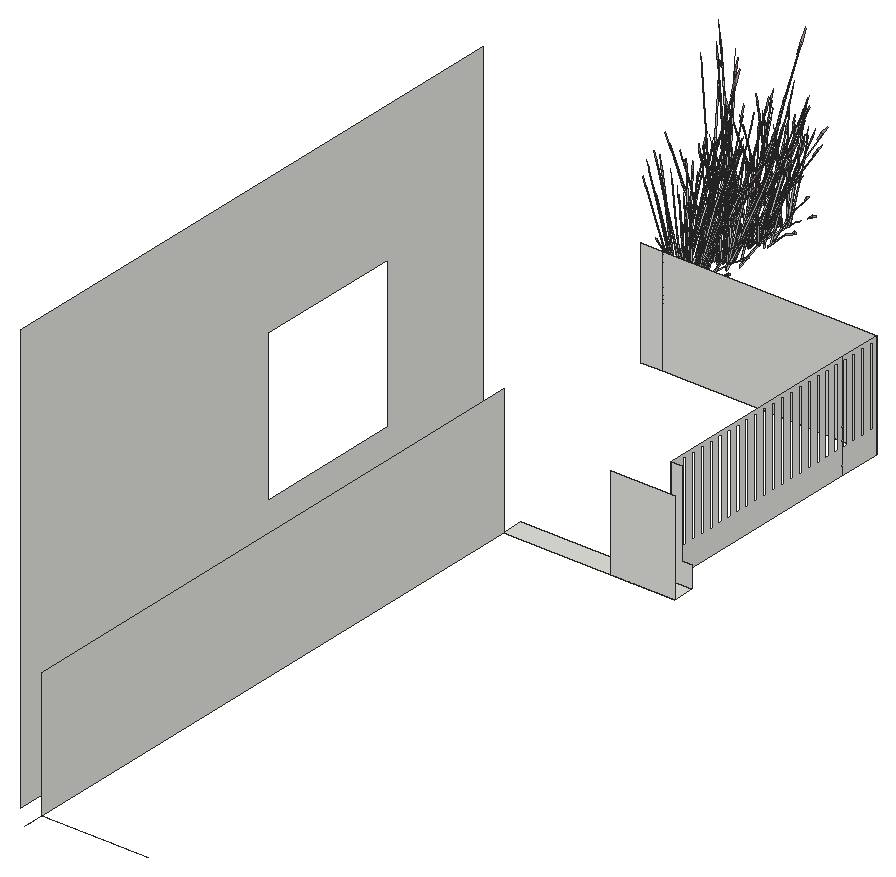
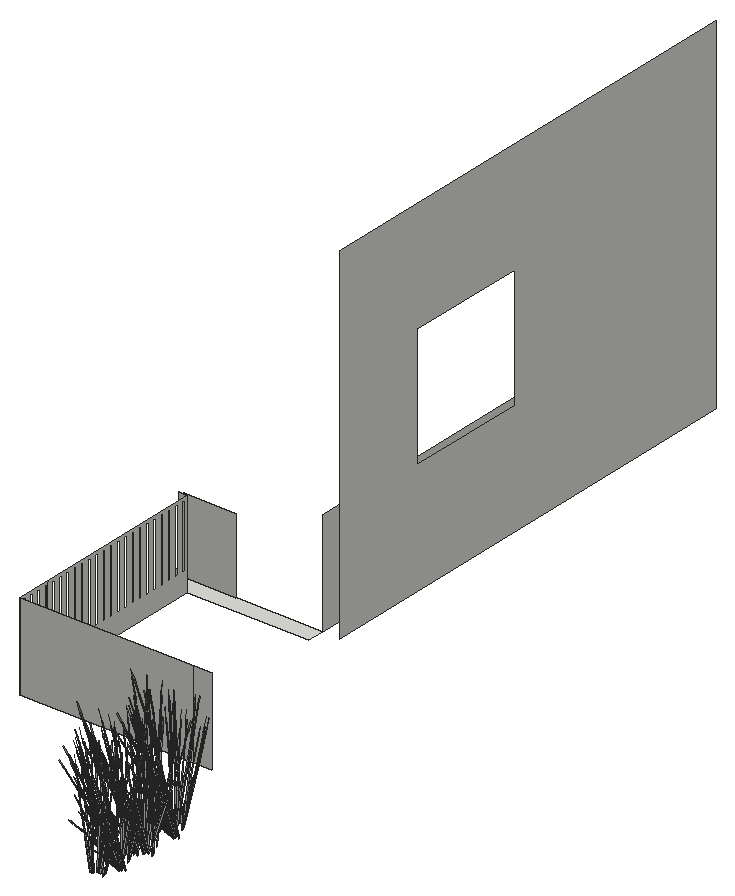
# SketchUp Ruby script. Lengths in inches.
U = 1.inch
M = Sketchup.active_model
def pt(a) = Geom::Point3d.new(a.map { |v| v * U })
def face(e, loops, mat)
  f = e.add_face(loops[0].map { |a| pt(a) })
  loops[1..].each { |l| e.add_face(l.map { |a| pt(a) }).erase! }
  f.material = f.back_material = mat if mat
  f
end
# faces: each face lists its corners as indices into pts; further lists are holes
def faces(e, pts, list, mat = nil) = list.each { |f| face(e, (f[0].is_a?(Array) ? f : [f]).map { |l| l.map { |i| pts[i] } }, mat) }
# xy, xz, yz: faces in a plane at the given z, y or x. An outline is a flat list of corners, or four numbers for a rectangle; further outlines are holes
def ring(l) = l.size == 4 ? [[l[0], l[1]], [l[2], l[1]], [l[2], l[3]], [l[0], l[3]]] : l.each_slice(2).to_a
def flat(e, list, mat, &to3) = list.each { |f| face(e, (f[0].is_a?(Array) ? f : [f]).map { |l| ring(l).map { |u, v| to3.(u, v) } }, mat) }
def xy(e, z, list, mat = nil) = flat(e, list, mat) { |x, y| [x, y, z] }
def xz(e, y, list, mat = nil) = flat(e, list, mat) { |x, z| [x, y, z] }
def yz(e, x, list, mat = nil) = flat(e, list, mat) { |y, z| [x, y, z] }
def lines(e, pts, list) = list.each { |a, b| e.add_line(pt(pts[a]), pt(pts[b])) }
# prism: a flat outline (further loops are holes) pulled along v
def prism(e, loops, v, mat = nil)
  f = face(e, loops, mat); d = Geom::Vector3d.new(v.map { |x| x * U })
  f.pushpull(f.normal.samedirection?(d) ? d.length : -d.length)
end
def box(e, o, s, mat = nil) = prism(e, [[o, [o[0] + s[0], o[1], o[2]], [o[0] + s[0], o[1] + s[1], o[2]], [o[0], o[1] + s[1], o[2]]]], [0, 0, s[2]], mat)
def at(x, y, z, deg = 0) = Geom::Transformation.translation(pt([x, y, z])) * Geom::Transformation.rotation(ORIGIN, Z_AXIS, deg.degrees)
def axes(o, x, y, z) = Geom::Transformation.new([*x, 0, *y, 0, *z, 0, *pt(o).to_a, 1])
def part(name) = M.definitions.add(name)
# library, detail: a bought-in or finely detailed component or shape, given as its bounding box
def library(name, o, s) = part(name).tap { |d| box(d.entities, o, s) }
def detail(e, o, s) = box(e.add_group.entities, o, s)
def put(e, d, t, mat = nil) = e.add_instance(d, t).tap { |i| i.material = mat if mat }
def group(e, t, mat = nil) = e.add_group.tap { |g| g.transformation = t; g.material = mat if mat }.entities
root = M.entities
M.materials.add("LightPink_Translucent").color = [144, 107, 117]
M.materials["LightPink_Translucent"].alpha = 0.75
c1 = part("blade")
p = [[2.15,0.21,22],[0,0.17,0],[0.09,0.45,0],[2.18,0.31,22],[2.29,0.31,22],[0.38,0.45,0],
  [2.48,0.24,33],[2.49,0.24,33],[2.48,0.22,33]]
faces(c1.entities,p,[[0,1,2,3],[4,5,2,3],[6,3,4,7],[8,0,3,6]])
c2 = part("seeds")
p = [[0.3,-0.1,1.38],[-0.01,-0.03,1.59],[-0.01,-0.03,0.03],[0.14,-0.07,-0.07],[0.29,-0.03,3],[0.15,0.01,3.11]]
faces(c2.entities,p,[[0,1,2,3],[1,0,4,5]],"LightPink_Translucent")
c3 = part("blade with seeds")
put(c3.entities,c1,at(0,0,0))
put(c3.entities,c2,axes([2.4,0.25,30.99],[1.5799,-0.05474,1.17369],[-0.12525,1.92788,0.29478],[-0.07173,-0.02425,1.56792]))
xy(root,126,[[312,213,360,219]])
xz(root,213,[[342,126,360,151.99]])
xz(root,219,[[354,126,354,156,357,156,357,132,360,132,360,126]])
xz(root,291,[[288,126,294,156],[294,126,354,156]])
yz(root,306,[[[51,126,213,246],[137.73,165,179.73,207]]])
yz(root,312,[[51,126,213,162]])
yz(root,354,[[[219,126,279,156],[220,133,221.125,155],[223.125,133,224.25,155],[226.25,133,227.375,155],[229.375,133,230.5,155],[232.5,133,233.625,155],[235.625,133,236.75,155],[238.75,133,239.875,155],[241.875,133,243,155],[245,133,246.125,155],[248.125,133,249.25,155],[251.25,133,252.375,155],[254.375,133,255.5,155],[257.5,133,258.625,155],[260.625,133,261.75,155],[263.75,133,264.875,155],[266.875,133,268,155],[270,133,271.125,155],[273.125,133,274.25,155],[276.25,133,277.375,155]],[[279,126,291,156],[279.375,133,280.5,155],[282.5,133,283.625,155],[285.625,133,286.75,155],[288.75,133,289.875,155]]])
p = [[312,51,126],[342,51,126],[312,45,126],[360,51,126],[360,45,126]]
lines(root,p,[[0,1],[0,2],[3,4]])
put(root,c3,axes([271,325.89,125.98],[-0.0219,-0.25042,1.71376],[0.94901,0.16613,0.13857],[-0.0587,0.35688,0.73262]))
put(root,c3,axes([271,338.87,126.89],[-0.0219,-0.25042,1.71376],[0.94901,0.16613,0.13857],[-0.0587,0.35688,0.73262]))
put(root,c3,axes([271,349.14,126.2],[-0.0219,-0.25042,1.71376],[0.94901,0.16613,0.13857],[-0.0587,0.35688,0.73262]))
put(root,c3,axes([271.51,337.65,125.73],[-0.43405,0.58792,0.44739],[-0.90188,-0.28295,-0.21531],[0,-0.13553,1.43643]))
put(root,c3,axes([272.94,334.82,127.99],[-0.42698,-0.53052,-0.71045],[0.87893,-0.29566,0.08574],[-0.09984,-0.25633,1.00501]))
put(root,c3,axes([272.94,355.63,127.625],[-0.42698,-0.53052,-0.71045],[0.87893,-0.29566,0.08574],[-0.09984,-0.25633,1.00501]))
put(root,c3,axes([273.11,321.92,127.16],[-0.2697,0.50175,0.35414],[-0.78684,-0.14635,-0.4572],[-0.07215,-0.20201,0.87481]))
put(root,c3,axes([271.4375,327.21,126.84],[-0.6592,0.22175,0.0643],[-0.32265,-0.40436,0.50621],[0.06366,0.17825,0.77189]))
put(root,c3,axes([271.4375,350.47,127.05],[-0.6592,0.22175,0.0643],[-0.32265,-0.40436,0.50621],[0.06366,0.17825,0.77189]))
put(root,c3,axes([273.6,337.92,125.73],[0.97146,-0.04028,0.44739],[0.08785,0.66859,-0.21531],[-0.17391,0.06776,1.43643]))
put(root,c3,axes([274.32,339.41,125.49],[0.83726,-0.32623,0.49651],[0.50045,0.58498,0],[-0.19069,0.0743,1.57504]))
put(root,c3,axes([273.02,321.39,126.63],[0.2697,-0.50175,-0.35414],[0.78684,0.14635,0.4572],[-0.07215,-0.20201,0.87481]))
put(root,c3,axes([273.02,334.37,127.54],[0.2697,-0.50175,-0.35414],[0.78684,0.14635,0.4572],[-0.07215,-0.20201,0.87481]))
put(root,c3,axes([273.02,344.64,126.85],[0.2697,-0.50175,-0.35414],[0.78684,0.14635,0.4572],[-0.07215,-0.20201,0.87481]))
put(root,c3,axes([273.02,355.18,127.17],[0.2697,-0.50175,-0.35414],[0.78684,0.14635,0.4572],[-0.07215,-0.20201,0.87481]))
put(root,c3,axes([271.77,327.29,126.63],[-0.2697,0.50175,-0.35414],[-0.78684,-0.14635,0.4572],[0.07215,0.20201,0.87481]))
put(root,c3,axes([271.77,340.26,127.54],[-0.2697,0.50175,-0.35414],[-0.78684,-0.14635,0.4572],[0.07215,0.20201,0.87481]))
put(root,c3,axes([271.77,350.54,126.85],[-0.2697,0.50175,-0.35414],[-0.78684,-0.14635,0.4572],[0.07215,0.20201,0.87481]))
put(root,c3,axes([273.35,321.46,126.84],[0.6592,-0.22175,0.0643],[0.32265,0.40436,0.50621],[-0.06366,-0.17825,0.77189]))
put(root,c3,axes([273.35,344.72,127.05],[0.6592,-0.22175,0.0643],[0.32265,0.40436,0.50621],[-0.06366,-0.17825,0.77189]))
put(root,c3,axes([271.21,328.18,126.82],[0.1134,0.10507,1.74944],[0.91515,0.04128,-0.27667],[0.09203,0.23172,0.14031]))
put(root,c3,axes([271.21,351.43,127.04],[0.1134,0.10507,1.74944],[0.91515,0.04128,-0.27667],[0.09203,0.23172,0.14031]))
put(root,c3,axes([273.12,321.51,126.84],[0.88151,0.17057,0.48003],[-0.30143,0.56078,0.3958],[-0.05297,-0.22053,0.9933]))
put(root,c3,axes([273.12,344.76,127.06],[0.88151,0.17057,0.48003],[-0.30143,0.56078,0.3958],[-0.05297,-0.22053,0.9933]))
put(root,c3,axes([271.74,336.83,125.73],[-0.97146,0.04028,0.44739],[-0.08785,-0.66859,-0.21531],[0.17391,-0.06776,1.43643]))
put(root,c3,axes([271.68,326.76,127.16],[0.2697,-0.50175,0.35414],[0.78684,0.14635,-0.4572],[0.07215,0.20201,0.87481]))
put(root,c3,axes([271.85,339.8125,127.99],[0.42698,0.53052,-0.71045],[-0.87893,0.29566,0.08574],[0.09984,0.25633,1.00501]))
put(root,c3,axes([273.16,333.31,125.78],[0.11476,0.38047,1.1486],[-0.63664,-0.21072,0.84392],[0.06851,-0.19481,0.25299]))
put(root,c3,axes([273.83,337.1,125.73],[0.43405,-0.58792,0.44739],[0.90188,0.28295,-0.21531],[0,0.13553,1.43643]))
put(root,c3,axes([272.17,339.92,127.69],[0.87941,0.16356,-0.51099],[-0.30143,0.56078,-0.3958],[0.08064,0.22578,0.97773]))
put(root,c3,axes([271.42,326.97,127.14],[0.87543,-0.30377,-0.1216],[0.4302,0.53915,-0.67495],[0.1155,0.2272,1.02557]))
put(root,c3,axes([271.42,350.22,127.36],[0.87543,-0.30377,-0.1216],[0.4302,0.53915,-0.67495],[0.1155,0.2272,1.02557]))
put(root,c3,axes([275.89,320.95,126.82],[-0.09085,0.04984,1.77383],[-0.89014,-0.16814,-0.16761],[-0.03222,-0.21748,0.31391]))
put(root,c3,axes([275.89,344.2,127.03],[-0.09085,0.04984,1.77383],[-0.89014,-0.16814,-0.16761],[-0.03222,-0.21748,0.31391]))
put(root,c3,axes([275.19,322.39,127.14],[-0.98321,-0.03233,-0.1216],[0.02687,-0.61208,-0.67495],[0.0683,-0.23574,1.02557]))
put(root,c3,axes([275.19,345.64,127.36],[-0.98321,-0.03233,-0.1216],[0.02687,-0.61208,-0.67495],[0.0683,-0.23574,1.02557]))
put(root,c3,axes([275.19,356.18,127.68],[-0.98321,-0.03233,-0.1216],[0.02687,-0.61208,-0.67495],[0.0683,-0.23574,1.02557]))
put(root,c3,axes([274.81,322.48,127.16],[-0.60531,0.34352,0.35414],[-0.573,-0.39225,-0.4572],[0.08718,-0.19929,0.87481]))
put(root,c3,axes([272.9,336.5625,125.73],[-0.53742,-0.54764,0.44739],[0.81403,-0.38564,-0.21531],[0.17391,0.06776,1.43643]))
put(root,c3,axes([274.52,335.14,127.69],[-0.64041,-0.4384,-0.51099],[0.67652,-0.38394,-0.3958],[0.09744,-0.22274,0.97773]))
put(root,c3,axes([274.52,355.95,127.33],[-0.64041,-0.4384,-0.51099],[0.67652,-0.38394,-0.3958],[0.09744,-0.22274,0.97773]))
put(root,c3,axes([273.87,327.04,126.84],[-0.88979,0.14973,0.48003],[-0.15442,-0.58737,0.3958],[0.20926,0.17311,0.9933]))
put(root,c3,axes([273.7,327.15,126.84],[-0.4066,0.41448,0.0643],[-0.57901,-0.24131,0.50621],[0.18719,0.13288,0.77189]))
put(root,c3,axes([273.7,350.4,127.05],[-0.4066,0.41448,0.0643],[-0.57901,-0.24131,0.50621],[0.18719,0.13288,0.77189]))
put(root,c3,axes([272.67,325.79,125.98],[-0.2045,-0.20949,1.71376],[0.94495,-0.17636,0.13857],[0.21357,0.32887,0.73262]))
put(root,c3,axes([272.67,338.76,126.89],[-0.2045,-0.20949,1.71376],[0.94495,-0.17636,0.13857],[0.21357,0.32887,0.73262]))
put(root,c3,axes([272.67,349.04,126.2],[-0.2045,-0.20949,1.71376],[0.94495,-0.17636,0.13857],[0.21357,0.32887,0.73262]))
put(root,c3,axes([274.72,335.34,127.99],[0.02328,-0.60353,-0.71045],[0.98022,0.04053,0.08574],[0.10344,-0.25568,1.00501]))
put(root,c3,axes([274.72,356.15,127.625],[0.02328,-0.60353,-0.71045],[0.98022,0.04053,0.08574],[0.10344,-0.25568,1.00501]))
put(root,c3,axes([273.57,326.68,127.16],[-0.13817,-0.52554,0.35414],[0.78985,-0.13877,-0.4572],[0.21215,0.1506,0.87481]))
put(root,c3,axes([274.1,323.65,126.58],[-0.77304,-0.33901,1.38283],[0.81626,-0.52782,0.59665],[0.24941,0.31809,1.33663]))
put(root,c3,axes([274.1,346.91,126.8],[-0.77304,-0.33901,1.38283],[0.81626,-0.52782,0.59665],[0.24941,0.31809,1.33663]))
put(root,c3,axes([275.12,322,126.63],[0.60531,-0.34352,-0.35414],[0.573,0.39225,0.4572],[0.08718,-0.19929,0.87481]))
put(root,c3,axes([275.12,334.97,127.54],[0.60531,-0.34352,-0.35414],[0.573,0.39225,0.4572],[0.08718,-0.19929,0.87481]))
put(root,c3,axes([275.12,345.25,126.85],[0.60531,-0.34352,-0.35414],[0.573,0.39225,0.4572],[0.08718,-0.19929,0.87481]))
put(root,c3,axes([275.12,355.78,127.17],[0.60531,-0.34352,-0.35414],[0.573,0.39225,0.4572],[0.08718,-0.19929,0.87481]))
put(root,c3,axes([272.8,327.41,126.82],[0.00265,-0.07899,1.77383],[0.76665,-0.34851,-0.16761],[0.2663,0.12439,0.31391]))
put(root,c3,axes([272.8,350.66,127.03],[0.00265,-0.07899,1.77383],[0.76665,-0.34851,-0.16761],[0.2663,0.12439,0.31391]))
put(root,c3,axes([275.36,322.17,126.84],[0.73517,0.0304,0.0643],[-0.02016,0.45906,0.50621],[0.07693,-0.17585,0.77189]))
put(root,c3,axes([275.36,345.43,127.05],[0.73517,0.0304,0.0643],[-0.02016,0.45906,0.50621],[0.07693,-0.17585,0.77189]))
put(root,c3,axes([275.27,339.39,125.78],[-0.5037,-0.18761,1.1486],[0.6504,-0.19062,0.84392],[0.17543,0.16147,0.25299]))
put(root,c3,axes([276.09,321.42,126.82],[-0.00864,-0.12985,1.74944],[-0.72937,-0.3753,-0.27667],[0.11277,-0.2275,0.14031]))
put(root,c3,axes([276.09,344.67,127.04],[-0.00864,-0.12985,1.74944],[-0.72937,-0.3753,-0.27667],[0.11277,-0.2275,0.14031]))
put(root,c3,axes([275.12,322.13,126.84],[0.63704,0.44518,0.48003],[-0.67652,0.38394,0.3958],[0.11751,-0.20886,0.9933]))
put(root,c3,axes([275.35,340.24,125.68],[-0.57368,-0.02046,1.0506],[0.37886,-0.43461,0.58006],[0.22663,0.15441,0.8241]))
put(root,c3,axes([275.86,323.55,127.16],[-0.77872,0.09325,0.35414],[-0.20563,-0.53305,-0.4572],[0.22316,-0.14318,0.87481]))
put(root,c3,axes([273.62,322.05,125.98],[-0.16657,0.22426,1.71376],[-0.69879,-0.4641,0.13857],[0.31524,-0.28926,0.73262]))
put(root,c3,axes([273.62,335.03,126.89],[-0.16657,0.22426,1.71376],[-0.69879,-0.4641,0.13857],[0.31524,-0.28926,0.73262]))
put(root,c3,axes([273.62,345.31,126.2],[-0.16657,0.22426,1.71376],[-0.69879,-0.4641,0.13857],[0.31524,-0.28926,0.73262]))
put(root,c3,axes([273.62,355.84,126.52],[-0.16657,0.22426,1.71376],[-0.69879,-0.4641,0.13857],[0.31524,-0.28926,0.73262]))
put(root,c3,axes([273.5,326.95,127.14],[0.53309,-0.55848,-0.1216],[0.77201,0.32175,-0.67495],[0.26836,0.15779,1.02557]))
put(root,c3,axes([273.5,350.2,127.36],[0.53309,-0.55848,-0.1216],[0.77201,0.32175,-0.67495],[0.26836,0.15779,1.02557]))
put(root,c3,axes([276.26,323.59,127.14],[-0.82753,-0.35977,-0.1216],[0.47675,-0.52101,-0.67495],[0.2338,-0.18111,1.02557]))
put(root,c3,axes([276.26,346.85,127.36],[-0.82753,-0.35977,-0.1216],[0.47675,-0.52101,-0.67495],[0.2338,-0.18111,1.02557]))
put(root,c3,axes([276.26,357.38,127.68],[-0.82753,-0.35977,-0.1216],[0.47675,-0.52101,-0.67495],[0.2338,-0.18111,1.02557]))
put(root,c3,axes([274.13,339.65,127.69],[0.88277,-0.1551,-0.51099],[0.15442,0.58737,-0.3958],[0.23711,0.16832,0.97773]))
put(root,c3,axes([275.14,325.97,127.16],[-0.50902,-0.40851,0.35414],[0.58122,-0.38671,-0.4572],[0.29531,0.05884,0.87481]))
put(root,c3,axes([275.61,326.34,126.84],[-0.04505,0.49615,0.0643],[-0.68022,-0.0136,0.50621],[0.26056,0.05192,0.77189]))
put(root,c3,axes([275.61,349.59,127.05],[-0.04505,0.49615,0.0643],[-0.68022,-0.0136,0.50621],[0.26056,0.05192,0.77189]))
put(root,c3,axes([275.67,326.18,126.84],[-0.65964,0.42992,0.48003],[-0.5689,-0.45657,0.3958],[0.30948,0.0793,0.9933]))
put(root,c3,axes([275.67,349.43,127.06],[-0.65964,0.42992,0.48003],[-0.5689,-0.45657,0.3958],[0.30948,0.0793,0.9933]))
put(root,c3,axes([275.85,336.15,127.69],[-0.22982,-0.59576,-0.51099],[0.87033,-0.10422,-0.3958],[0.24941,-0.16002,0.97773]))
put(root,c3,axes([275.85,356.96,127.33],[-0.22982,-0.59576,-0.51099],[0.87033,-0.10422,-0.3958],[0.24941,-0.16002,0.97773]))
put(root,c3,axes([277.38,326.24,126.04],[-0.17122,-0.54847,-0.03492],[0.80929,-0.12609,-0.15832],[0.169,0.03477,0.52218]))
put(root,c3,axes([277.38,339.22,126.94],[-0.17122,-0.54847,-0.03492],[0.80929,-0.12609,-0.15832],[0.169,0.03477,0.52218]))
put(root,c3,axes([277.38,349.5,126.25],[-0.17122,-0.54847,-0.03492],[0.80929,-0.12609,-0.15832],[0.169,0.03477,0.52218]))
put(root,c3,axes([275.98,324.82,127.16],[-0.74348,-0.18202,0.35414],[0.21685,-0.53102,-0.4572],[0.29933,-0.04869,0.87481]))
put(root,c3,axes([276.92,334.96,125.78],[-0.29798,0.33213,1.1486],[-0.25612,-0.44624,0.84392],[0.24611,-0.11182,0.25299]))
put(root,c3,axes([276.5625,323.46,126.84],[0.61415,0.2744,0.0643],[-0.35756,0.39076,0.50621],[0.1969,-0.12633,0.77189]))
put(root,c3,axes([276.5625,346.71,127.05],[0.61415,0.2744,0.0643],[-0.35756,0.39076,0.50621],[0.1969,-0.12633,0.77189]))
put(root,c3,axes([276.39,323.35,126.84],[0.22187,0.60049,0.48003],[-0.87033,0.10422,0.3958],[0.25651,-0.14123,0.9933]))
put(root,c3,axes([274.04,325.13,125.98],[-0.3323,-0.11241,1.71376],[0.68769,-0.4716,0.13857],[0.42861,0.21275,0.73262]))
put(root,c3,axes([274.04,338.11,126.89],[-0.3323,-0.11241,1.71376],[0.68769,-0.4716,0.13857],[0.42861,0.21275,0.73262]))
put(root,c3,axes([274.04,348.39,126.2],[-0.3323,-0.11241,1.71376],[0.68769,-0.4716,0.13857],[0.42861,0.21275,0.73262]))
put(root,c3,axes([278.3,323.4375,126.82],[-0.11685,-0.00496,1.77383],[-0.48522,-0.53096,-0.16761],[0.19486,-0.17458,0.31391]))
put(root,c3,axes([278.3,346.69,127.03],[-0.11685,-0.00496,1.77383],[-0.48522,-0.53096,-0.16761],[0.19486,-0.17458,0.31391]))
put(root,c3,axes([276.49,323.23,126.63],[0.77872,-0.09325,-0.35414],[0.20563,0.53305,0.4572],[0.22316,-0.14318,0.87481]))
put(root,c3,axes([276.49,336.21,127.54],[0.77872,-0.09325,-0.35414],[0.20563,0.53305,0.4572],[0.22316,-0.14318,0.87481]))
put(root,c3,axes([276.49,346.48,126.85],[0.77872,-0.09325,-0.35414],[0.20563,0.53305,0.4572],[0.22316,-0.14318,0.87481]))
put(root,c3,axes([276.49,357.02,127.17],[0.77872,-0.09325,-0.35414],[0.20563,0.53305,0.4572],[0.22316,-0.14318,0.87481]))
put(root,c3,axes([275.875,336.39,127.99],[0.4673,-0.51481,-0.71045],[0.81887,0.36587,0.08574],[0.27902,-0.18652,1.00501]))
put(root,c3,axes([275.875,357.2,127.625],[0.4673,-0.51481,-0.71045],[0.81887,0.36587,0.08574],[0.27902,-0.18652,1.00501]))
put(root,c3,axes([276.66,324.99,126.84],[0.32857,0.44488,0.0643],[-0.59916,0.21775,0.50621],[0.26412,-0.04296,0.77189]))
put(root,c3,axes([276.66,348.24,127.05],[0.32857,0.44488,0.0643],[-0.59916,0.21775,0.50621],[0.26412,-0.04296,0.77189]))
put(root,c3,axes([275.87,326.18,126.63],[0.50902,0.40851,-0.35414],[-0.58122,0.38671,0.4572],[0.29531,0.05884,0.87481]))
put(root,c3,axes([275.87,339.16,127.54],[0.50902,0.40851,-0.35414],[-0.58122,0.38671,0.4572],[0.29531,0.05884,0.87481]))
put(root,c3,axes([275.87,349.43,126.85],[0.50902,0.40851,-0.35414],[-0.58122,0.38671,0.4572],[0.29531,0.05884,0.87481]))
put(root,c3,axes([275.28,326.23,127.14],[0.0479,-0.66354,-0.1216],[0.90696,0.01814,-0.67495],[0.3493,0.04609,1.02557]))
put(root,c3,axes([275.28,349.48,127.36],[0.0479,-0.66354,-0.1216],[0.90696,0.01814,-0.67495],[0.3493,0.04609,1.02557]))
put(root,c3,axes([276.29,325,127.14],[-0.45012,-0.59081,-0.1216],[0.79888,-0.29033,-0.67495],[0.33665,-0.07795,1.02557]))
put(root,c3,axes([276.29,348.25,127.36],[-0.45012,-0.59081,-0.1216],[0.79888,-0.29033,-0.67495],[0.33665,-0.07795,1.02557]))
put(root,c3,axes([276.59,324.83,126.84],[-0.25275,0.59491,0.48003],[-0.83094,-0.20343,0.3958],[0.32677,-0.03575,0.9933]))
put(root,c3,axes([276.59,348.08,127.06],[-0.25275,0.59491,0.48003],[-0.83094,-0.20343,0.3958],[0.32677,-0.03575,0.9933]))
put(root,c3,axes([276.07,325.83,126.82],[0.19191,-0.01103,1.74944],[0.52639,-0.5069,-0.27667],[0.34136,0.06691,0.14031]))
put(root,c3,axes([276.07,349.08,127.04],[0.19191,-0.01103,1.74944],[0.52639,-0.5069,-0.27667],[0.34136,0.06691,0.14031]))
put(root,c3,axes([276.26,337.47,127.69],[0.24236,-0.59349,-0.51099],[0.83094,0.20343,-0.3958],[0.33455,-0.05442,0.97773]))
put(root,c3,axes([278.34,337.85,125.78],[-0.55274,0.10771,1.1486],[0.26018,-0.44517,0.84392],[0.29323,0.03046,0.25299]))
put(root,c3,axes([276.76,324.76,126.63],[0.74348,0.18202,-0.35414],[-0.21685,0.53102,0.4572],[0.29933,-0.04869,0.87481]))
put(root,c3,axes([276.76,337.74,127.54],[0.74348,0.18202,-0.35414],[-0.21685,0.53102,0.4572],[0.29933,-0.04869,0.87481]))
put(root,c3,axes([276.76,348.01,126.85],[0.74348,0.18202,-0.35414],[-0.21685,0.53102,0.4572],[0.29933,-0.04869,0.87481]))
put(root,c3,axes([275.33,338.88,127.99],[0.89428,0.01571,-0.71045],[-0.06006,0.66153,0.08574],[0.37886,0.06981,1.00501]))
put(root,c3,axes([278.09,326.75,126.82],[-0.08089,-0.05712,1.77383],[0.17695,-0.61228,-0.16761],[0.31864,-0.03912,0.31391]))
put(root,c3,axes([278.09,350.01,127.03],[-0.08089,-0.05712,1.77383],[0.17695,-0.61228,-0.16761],[0.31864,-0.03912,0.31391]))
put(root,c3,axes([274.74,324.1,125.98],[-0.37107,0.01478,1.71376],[0.24616,-0.64047,0.13857],[0.5288,0.03961,0.73262]))
put(root,c3,axes([274.74,337.08,126.89],[-0.37107,0.01478,1.71376],[0.24616,-0.64047,0.13857],[0.5288,0.03961,0.73262]))
put(root,c3,axes([274.74,347.36,126.2],[-0.37107,0.01478,1.71376],[0.24616,-0.64047,0.13857],[0.5288,0.03961,0.73262]))
put(root,c3,axes([276.1,337.68,127.99],[0.78611,-0.28816,-0.71045],[0.4381,0.59317,0.08574],[0.37982,-0.06738,1.00501]))
put(root,c3,axes([278.74,324.07,126.82],[0.12414,-0.09938,1.74944],[-0.15889,-0.60963,-0.27667],[0.31148,-0.11559,0.14031]))
put(root,c3,axes([278.74,347.33,127.04],[0.12414,-0.09938,1.74944],[-0.15889,-0.60963,-0.27667],[0.31148,-0.11559,0.14031]))
